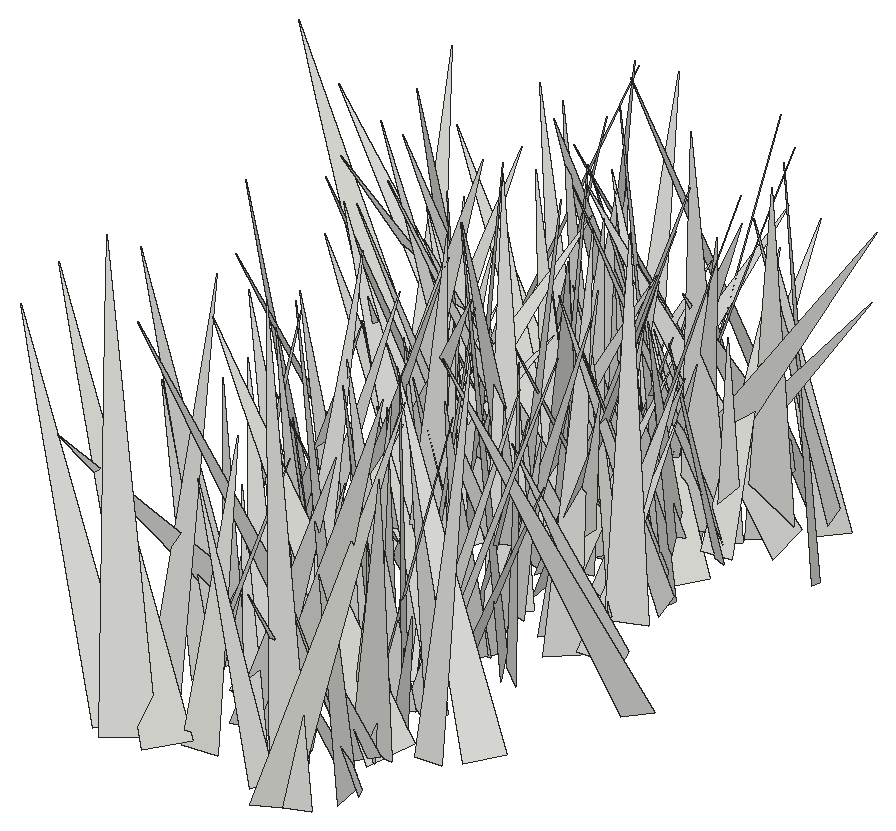
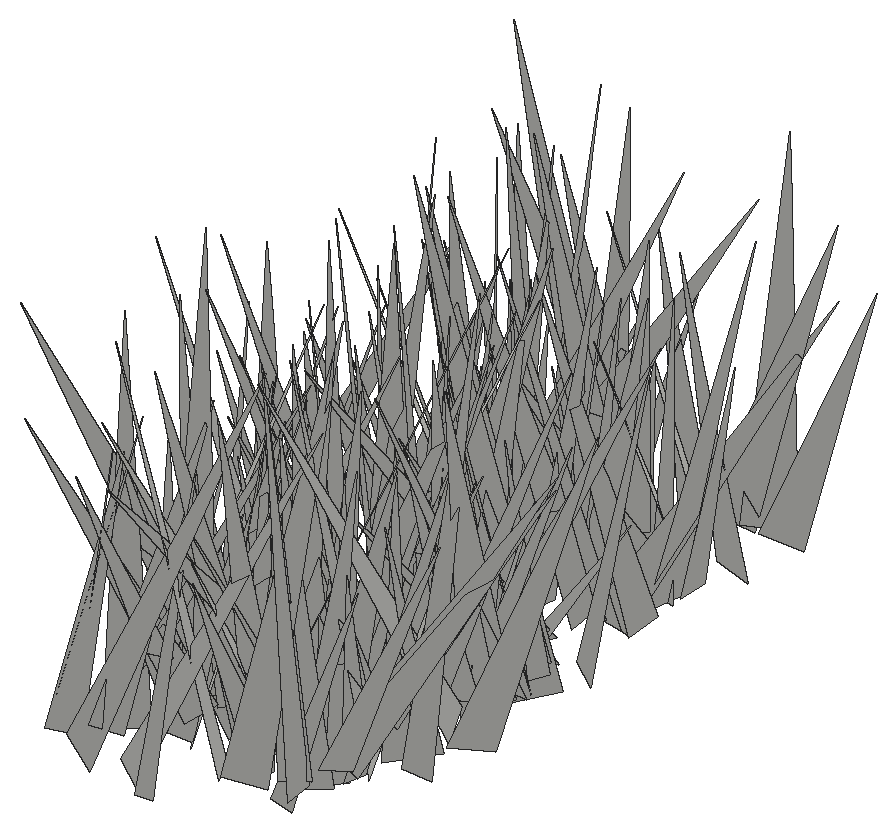
# SketchUp Ruby script. Lengths in inches.
U = 1.inch
M = Sketchup.active_model
def pt(a) = Geom::Point3d.new(a.map { |v| v * U })
def face(e, loops, mat)
  f = e.add_face(loops[0].map { |a| pt(a) })
  loops[1..].each { |l| e.add_face(l.map { |a| pt(a) }).erase! }
  f.material = f.back_material = mat if mat
  f
end
# faces: each face lists its corners as indices into pts; further lists are holes
def faces(e, pts, list, mat = nil) = list.each { |f| face(e, (f[0].is_a?(Array) ? f : [f]).map { |l| l.map { |i| pts[i] } }, mat) }
# xy, xz, yz: faces in a plane at the given z, y or x. An outline is a flat list of corners, or four numbers for a rectangle; further outlines are holes
def ring(l) = l.size == 4 ? [[l[0], l[1]], [l[2], l[1]], [l[2], l[3]], [l[0], l[3]]] : l.each_slice(2).to_a
def flat(e, list, mat, &to3) = list.each { |f| face(e, (f[0].is_a?(Array) ? f : [f]).map { |l| ring(l).map { |u, v| to3.(u, v) } }, mat) }
def xy(e, z, list, mat = nil) = flat(e, list, mat) { |x, y| [x, y, z] }
def xz(e, y, list, mat = nil) = flat(e, list, mat) { |x, z| [x, y, z] }
def yz(e, x, list, mat = nil) = flat(e, list, mat) { |y, z| [x, y, z] }
def lines(e, pts, list) = list.each { |a, b| e.add_line(pt(pts[a]), pt(pts[b])) }
# prism: a flat outline (further loops are holes) pulled along v
def prism(e, loops, v, mat = nil)
  f = face(e, loops, mat); d = Geom::Vector3d.new(v.map { |x| x * U })
  f.pushpull(f.normal.samedirection?(d) ? d.length : -d.length)
end
def box(e, o, s, mat = nil) = prism(e, [[o, [o[0] + s[0], o[1], o[2]], [o[0] + s[0], o[1] + s[1], o[2]], [o[0], o[1] + s[1], o[2]]]], [0, 0, s[2]], mat)
def at(x, y, z, deg = 0) = Geom::Transformation.translation(pt([x, y, z])) * Geom::Transformation.rotation(ORIGIN, Z_AXIS, deg.degrees)
def axes(o, x, y, z) = Geom::Transformation.new([*x, 0, *y, 0, *z, 0, *pt(o).to_a, 1])
def part(name) = M.definitions.add(name)
# library, detail: a bought-in or finely detailed component or shape, given as its bounding box
def library(name, o, s) = part(name).tap { |d| box(d.entities, o, s) }
def detail(e, o, s) = box(e.add_group.entities, o, s)
def put(e, d, t, mat = nil) = e.add_instance(d, t).tap { |i| i.material = mat if mat }
def group(e, t, mat = nil) = e.add_group.tap { |g| g.transformation = t; g.material = mat if mat }.entities
root = M.entities
c1 = part("fur_instance\#9")
p = [[0.8125,0,1.79],[0.67,-0.02,1.48],[0,-0.11,0],[0,0.11,0]]
faces(c1.entities,p,[[0,1,2,3]])
put(root,c1,axes([64.62,188,-27.1],[-5.80896,4.38047,0.69826],[4.41604,5.60261,1.59041],[-0.41794,-1.68592,7.09952]))
put(root,c1,axes([64.88,182.09,-27.1],[-3.28868,-4.79968,1.75844],[-5.10998,3.14053,-0.98472],[0.13097,2.01112,5.73434]))
put(root,c1,axes([66.55,170.2,-28.22],[-3.24359,5.98487,0.42852],[5.75195,2.96279,2.1587],[-1.708,-1.38792,6.45597]))
put(root,c1,axes([67.98,188.64,-27.1],[-5.05806,4.73106,0.08976],[4.36112,4.60989,2.7757],[-1.83619,-2.08349,6.34527]))
put(root,c1,axes([67.13,191.16,-27.1],[-0.73144,-5.99959,0.26703],[-5.39662,0.53861,-2.681],[-2.63493,0.56233,5.41685]))
put(root,c1,axes([67.08,191.65,-27.1],[-4.48303,2.72425,0.35571],[2.72908,4.33728,1.17718],[-0.3165,-1.18832,5.11208]))
put(root,c1,axes([66.97,175.47,-28.22],[-7.08698,0.49693,1.41438],[0.58095,7.2106,0.37757],[1.38199,-0.48283,7.09434]))
put(root,c1,axes([67.08,184.73,-27.1],[-4.89818,0.93846,0.55806],[1.01529,4.8584,0.74127],[0.40164,-0.83642,4.93188]))
put(root,c1,axes([68.67,170.12,-28.22],[-3.17251,7.14398,0.8627],[6.87917,2.73438,2.65436],[-2.11131,-1.82544,7.35225]))
put(root,c1,axes([66.78,174.3,-28.22],[-4.79431,0.50788,0.77321],[0.45097,4.84644,-0.38709],[0.80772,0.30866,4.80557]))
put(root,c1,axes([64.93,190.31,-27.1],[-2.27672,-7.40144,1.23154],[-7.29478,2.48469,1.44709],[1.75622,0.72557,7.60728]))
put(root,c1,axes([67.08,184.07,-28.22],[-6.50457,4.89284,0.5628],[4.72218,6.46057,-1.59001],[1.39918,0.94188,7.98255]))
put(root,c1,axes([67.36,186.7,-27.1],[-2.8111,-5.64649,0.53318],[-5.64839,2.7334,-0.83291],[-0.51273,0.84565,6.25232]))
put(root,c1,axes([68.09,181.38,-28.22],[-2.80536,-2.90649,0.0794],[-2.63209,2.49174,-1.78533],[-1.23535,1.29136,3.62358]))
put(root,c1,axes([67.5625,177.47,-28.22],[3.04305,-5.48081,0.27728],[-4.42438,-2.6378,-3.58374],[-3.24669,-1.54241,5.14356]))
put(root,c1,axes([67.4,169.73,-28.22],[-4.19179,6.94453,1.88873],[7.18228,4.17546,0.58769],[0.45687,-1.92457,8.09026]))
put(root,c1,axes([66.57,172.59,-28.22],[1.29784,6.7007,1.25957],[6.74597,-1.44798,0.75208],[-0.98888,-1.08363,6.78367]))
put(root,c1,axes([68.74,182.58,-28.22],[-2.83632,-6.0499,0.28173],[-5.90232,2.69141,-1.62612],[-1.35766,0.93829,6.48088]))
put(root,c1,axes([65.36,189.05,-27.1],[1.8239,-3.22944,0.77362],[-3.28665,-1.6292,0.94764],[0.47508,1.1273,3.58579]))
put(root,c1,axes([67.39,189.66,-28.22],[-3.97352,-3.33663,0.47318],[-3.25036,3.98768,0.8243],[0.89005,-0.33346,5.12275]))
put(root,c1,axes([67.52,190.17,-28.22],[-7.05336,-2.15617,1.71578],[-1.62887,7.06566,2.18314],[2.22256,-1.66441,7.04506]))
put(root,c1,axes([68.26,182.66,-27.1],[-3.16034,-1.96863,0.75138],[-2.10046,2.8354,-1.40585],[-0.16774,1.5852,3.44773]))
put(root,c1,axes([65.91,184.37,-27.1],[1.29367,6.30142,0.29631],[6.29029,-1.26564,-0.54746],[0.47747,-0.39942,6.4095]))
put(root,c1,axes([65.85,183.12,-27.1],[3.70802,-0.97097,0.29213],[-0.94384,-3.70994,-0.3508],[-0.37053,-0.26665,3.81695]))
put(root,c1,axes([67.24,175.28,-28.22],[1.09401,4.63876,2.44173],[5.21296,-1.22556,-0.00737],[-0.55243,-2.37843,4.76601]))
put(root,c1,axes([67.91,173.31,-28.22],[3.80784,5.11048,0.67094],[4.57882,-3.73693,2.47721],[-2.36675,0.99257,5.87197]))
put(root,c1,axes([68.39,189.01,-28.22],[-4.24883,1.88722,0.42776],[1.75815,4.19597,-1.04876],[0.80838,0.79335,4.52927]))
put(root,c1,axes([66.7,185.7,-27.1],[1.07751,-3.9043,2.33703],[-4.53898,-0.75293,0.83488],[0.32078,2.46086,3.96327]))
put(root,c1,axes([68.27,192.88,-28.22],[-0.08918,-3.86635,0.81214],[-3.84672,-0.10019,-0.89937],[-0.90053,0.81086,3.76135]))
put(root,c1,axes([68.89,176.65,-28.22],[-2.59565,5.50063,1.7013],[5.74289,2.3395,1.19781],[-0.41302,-2.03926,5.96319]))
put(root,c1,axes([65.99,187.07,-27.1],[6.85876,3.23862,0.41321],[3.02392,-6.66397,2.03701],[-1.23097,1.67477,7.30628]))
put(root,c1,axes([69.88,189.02,-28.22],[-6.64184,2.29308,0.28161],[2.23011,6.58737,-1.04152],[0.60342,0.8944,6.94892]))
put(root,c1,axes([67.77,188.22,-28.22],[1.11267,-4.69864,0.20362],[-4.67497,-1.12782,-0.47895],[-0.51316,0.0867,4.80478]))
put(root,c1,axes([69.62,184.96,-27.1],[-4.99004,2.24313,0.58277],[2.2784,5.00139,0.2583],[0.42444,-0.4756,5.46492]))
put(root,c1,axes([68.89,185,-27.1],[-3.32365,-1.7064,1.24939],[-2.04417,3.18881,-1.08271],[0.54234,1.56176,3.57578]))
put(root,c1,axes([67.33,184.88,-27.1],[4.65411,-4.15615,0.09318],[-4.0063,-4.52139,-1.56511],[-1.10988,-1.10744,6.04026]))
put(root,c1,axes([67.25,188.45,-28.22],[4.72712,-1.54603,0.79765],[-1.39638,-4.74943,-0.93014],[-1.03759,-0.65178,4.88576]))
put(root,c1,axes([66.54,177.04,-28.22],[6.22243,-0.20354,0.93497],[-0.30289,-6.25415,0.65425],[-0.90767,0.69164,6.19128]))
put(root,c1,axes([69.18,176.63,-28.22],[4.90342,0.51596,3.18153],[0.4361,-5.84514,0.27581],[-3.19346,-0.00597,4.92277]))
put(root,c1,axes([67.07,193.55,-27.1],[6.76883,1.43904,1.95286],[1.74836,-6.90673,-0.9705],[-1.68159,-1.38844,6.85171]))
put(root,c1,axes([66.41,183.87,-27.1],[-0.23722,4.19444,0.05409],[3.55446,0.22976,-2.22834],[2.22756,0.08005,3.56147]))
put(root,c1,axes([67.0625,182.21,-28.22],[3.97347,4.57155,1.31094],[4.73936,-3.94824,-0.59665],[-0.39506,-1.38509,6.02757]))
put(root,c1,axes([71.19,183.9,-27.1],[-7.48937,-0.81173,0.36322],[-0.84224,7.4632,-0.68756],[0.28542,0.72333,7.50179]))
put(root,c1,axes([67.51,180.82,-28.22],[-0.63862,5.35473,0.03552],[5.1577,0.62471,-1.44573],[1.43964,0.13724,5.19527]))
put(root,c1,axes([67.02,189.9375,-27.1],[6.14666,2.4589,1.36982],[2.59506,-6.2248,-0.47069],[-1.09008,-0.95377,6.60349]))
put(root,c1,axes([69.4,183.05,-27.1],[-4.06626,4.25963,1.22614],[4.27905,4.20638,-0.4224],[1.15655,-0.5867,5.87371]))
put(root,c1,axes([69.06,184.62,-28.22],[-4.34525,-4.69158,2.51984],[-5.05188,4.66036,-0.03462],[1.68493,1.87398,6.3946]))
put(root,c1,axes([67.78,190.75,-28.22],[4.73789,-1.18845,0.72275],[-0.9672,-4.65874,-1.32025],[-0.99966,-1.12521,4.70287]))
put(root,c1,axes([70.86,186.67,-28.22],[-3.00084,5.06154,0.45444],[5.0055,2.85272,1.2797],[-0.87785,-1.03611,5.74339]))
put(root,c1,axes([69.875,178.06,-28.22],[-6.22894,0.57755,1.75246],[0.68588,6.45268,0.31131],[1.71297,-0.48351,6.24791]))
put(root,c1,axes([67.48,177.55,-28.22],[2.77668,6.00015,1.42785],[6.14966,-2.57364,-1.14395],[0.47149,-1.76779,6.51177]))
put(root,c1,axes([66.7,182.66,-27.1],[0.11593,7.32982,3.76994],[7.80213,1.11829,-2.4142],[2.6581,-3.60212,6.9218]))
put(root,c1,axes([70.47,187.62,-27.1],[2.04194,-5.37013,1.21962],[-4.97283,-2.35693,-2.05211],[-2.36574,0.31918,5.36625]))
put(root,c1,axes([67.66,192.96,-27.1],[0.9975,-5.62203,0.93729],[-5.55991,-0.75041,1.41599],[1.25425,1.14473,5.53148]))
put(root,c1,axes([68.82,194.03,-27.1],[1.6119,-7.35068,0.1441],[-7.34568,-1.61634,-0.28263],[-0.30696,0.08011,7.52003]))
put(root,c1,axes([68.14,191.46,-28.22],[2.75053,-5.09352,1.52718],[-5.31748,-2.64324,0.76119],[-0.02665,1.70616,5.73847]))
put(root,c1,axes([70.69,185.05,-28.22],[-0.44719,-4.16584,0.88919],[-4.01944,0.11666,-1.47491],[-1.41032,0.98845,3.92158]))
put(root,c1,axes([69.04,176.18,-28.22],[-1.25475,3.57203,1.31412],[3.70812,1.4592,-0.42579],[0.858,-1.08261,3.76198]))
put(root,c1,axes([67.28,181.39,-27.1],[-1.44675,6.62808,0.1342],[5.91861,1.35324,-3.03008],[2.98656,0.529,6.06986]))
put(root,c1,axes([68.09,185.27,-28.22],[3.1539,-2.32332,0.00557],[-2.32207,-3.15188,0.13648],[0.07647,0.11319,3.91488]))
put(root,c1,axes([70.49,172.875,-28.22],[3.00603,-4.02582,3.59921],[-4.80148,-3.87769,-0.32715],[-2.47129,2.63706,5.01362]))
put(root,c1,axes([70.3125,186.72,-28.22],[-1.93771,-4.14246,0.35212],[-4.15628,1.93921,-0.05843],[0.0961,0.34375,4.57288]))
put(root,c1,axes([72.51,182.65,-27.1],[-6.31151,-2.93767,0.11387],[-2.9284,6.25835,-0.85765],[-0.25951,0.82534,6.90866]))
put(root,c1,axes([69.65,170.5,-28.22],[-1.16882,5.10436,1.64073],[5.31118,1.33199,-0.3603],[0.7334,-1.51127,5.22406]))
put(root,c1,axes([71.24,171.35,-28.22],[-0.27528,4.26527,0.41219],[4.05575,0.12601,1.40472],[-1.38323,-0.47937,4.03672]))
put(root,c1,axes([71.03,186.8125,-27.1],[-1.86081,5.49202,1.44787],[5.66351,1.67938,0.90859],[-0.42807,-1.65488,5.72707]))
put(root,c1,axes([68.9375,176.53,-28.22],[1.7878,3.1828,1.34143],[3.44443,-1.53093,-0.95817],[0.2561,-1.62848,3.52255]))
put(root,c1,axes([74.05,173.3125,-28.22],[-3.051,-7.21191,1.32168],[-6.61753,2.09219,-3.8598],[-3.15701,2.58422,6.81338]))
put(root,c1,axes([72.47,179.52,-28.22],[-6.11884,4.72961,1.11538],[4.85918,5.97068,1.339],[0.0418,-1.7422,7.61686]))
put(root,c1,axes([68.74,173.93,-28.22],[-1.28039,5.01222,0.36244],[4.5705,1.31696,-2.06622],[2.08908,0.19072,4.74262]))
put(root,c1,axes([70.63,180.96,-28.22],[-4.7564,-0.43454,1.78324],[-0.95829,4.81251,-1.3833],[1.56539,1.62573,4.5715]))
put(root,c1,axes([66.38,182.54,-28.22],[3.10816,-7.62871,0.22312],[-7.12075,-2.81203,3.04879],[2.74626,1.34273,7.65263]))
put(root,c1,axes([70.68,175.83,-28.22],[3.31439,2.62679,2.62231],[3.03004,-3.94532,0.12232],[-2.14367,-1.5153,4.22732]))
put(root,c1,axes([69.23,184.2,-28.22],[6.90611,3.10223,2.59996],[3.46907,-7.18559,-0.64093],[-2.08547,-1.6797,7.5437]))
put(root,c1,axes([68.28,171.6,-28.22],[4.70564,3.18962,0.73071],[3.27223,-4.59158,-1.02983],[-0.01227,-1.26267,5.59072]))
put(root,c1,axes([68.32,177.56,-28.22],[7.58645,0.4489,1.20084],[0.2907,-7.62155,1.01257],[-1.24861,0.95304,7.53196]))
put(root,c1,axes([70.88,190.52,-27.1],[-0.70792,6.63222,0.94241],[6.69223,0.65809,0.39581],[-0.29764,-0.97786,6.65814]))
put(root,c1,axes([72.08,187.16,-27.1],[-6.95078,-0.2098,1.40903],[-0.48679,6.94525,-1.36721],[1.33881,1.43604,6.81821]))
put(root,c1,axes([70.14,191.64,-28.22],[3.6116,-2.54944,1.03868],[-2.46348,-3.75778,-0.65768],[-1.22872,0.0404,4.37159]))
put(root,c1,axes([70.62,190.91,-28.22],[-2.94733,3.27814,0.42411],[3.06608,2.92358,-1.29021],[1.23501,0.56503,4.21525]))
put(root,c1,axes([68.83,190.6,-27.1],[1.67584,3.97009,0.12724],[3.80521,-1.56498,-1.28741],[1.13936,-0.61275,4.1125]))
put(root,c1,axes([72.51,170.03,-28.22],[-4.9286,0.63717,0.02707],[0.62924,4.89286,-0.60144],[0.10377,0.59304,4.93308]))
put(root,c1,axes([71.65,180.29,-28.22],[0.78619,5.10987,0.99795],[4.99569,-1.02461,1.31074],[-1.46621,-0.75112,5.00108]))
put(root,c1,axes([73.25,185.13,-27.1],[-6.90561,-3.33755,0.10935],[-3.32242,6.89219,0.54573],[0.33571,-0.44394,7.65042]))
put(root,c1,axes([73.2,194.27,-28.22],[-3.69679,-5.87263,0.02895],[-5.78236,3.6339,-1.23044],[-1.02613,0.67962,6.82936]))
put(root,c1,axes([71.11,177.5625,-28.22],[-3.39336,2.50243,2.08506],[2.97495,3.60715,0.51243],[1.32637,-1.68843,4.18502]))
put(root,c1,axes([71.59,190.17,-28.22],[-4.44345,-1.97155,1.25823],[-1.71315,4.58269,1.13072],[1.59225,-0.57131,4.72787]))
put(root,c1,axes([71.38,189.24,-28.22],[3.36886,3.17868,0.5186],[2.75759,-3.23451,1.91201],[-1.66392,1.0752,4.2187]))
put(root,c1,axes([74.49,173.95,-28.22],[-6.95314,3.37085,0.59923],[3.40426,6.66259,2.02209],[-0.36434,-2.07731,7.45788]))
put(root,c1,axes([68.25,187.45,-28.22],[3.98085,5.13777,1.04709],[4.9615,-3.26572,-2.83883],[1.69606,-2.50573,5.84679]))
put(root,c1,axes([70.56,186.32,-28.22],[-0.53064,3.51066,0.60828],[3.36851,0.69471,-1.0709],[1.16098,-0.41106,3.38519]))
put(root,c1,axes([73.09,178.31,-28.22],[-4.19942,1.95994,0.17006],[1.96728,4.18576,0.33862],[0.01038,-0.37878,4.62189]))
put(root,c1,axes([70.54,188.29,-28.22],[3.92094,-4.8226,1.73149],[-5.06492,-3.97791,0.39007],[-0.77596,1.59628,6.20315]))
put(root,c1,axes([71.25,186.01,-28.22],[4.78863,4.89843,2.46119],[5.13986,-5.14824,0.24599],[-1.90629,-1.57608,6.84581]))
put(root,c1,axes([72.375,178.27,-28.22],[-2.92778,3.00983,0.00711],[2.98882,2.90849,-0.48849],[0.35507,0.33555,4.17041]))
put(root,c1,axes([73.11,191.22,-28.22],[-5.49942,-3.45806,0.94275],[-3.51329,5.5426,-0.16378],[0.70973,0.64178,6.49422]))
put(root,c1,axes([71.97,189.28,-27.1],[2.76185,-3.07557,2.49035],[-3.57907,-3.23702,-0.02845],[-1.68858,1.83068,4.13354]))
put(root,c1,axes([70.5,189.77,-27.1],[2.46707,-3.42013,1.11602],[-3.59628,-2.30764,0.87798],[0.09798,1.4166,4.12467]))
put(root,c1,axes([71.31,184.68,-27.1],[-1.28259,-7.19659,1.19017],[-7.23451,1.40948,0.72639],[0.93233,1.03678,7.27381]))
put(root,c1,axes([71.2,179.47,-28.22],[6.01123,-4.10409,2.83515],[-4.50522,-6.3728,0.32708],[-2.14119,1.8869,7.27128]))
put(root,c1,axes([72.04,181.125,-28.22],[-1.26664,-5.03308,1.07763],[-5.14261,1.28411,-0.04714],[0.2163,1.05675,5.1898]))
put(root,c1,axes([72.18,171.66,-28.22],[0.64716,8.27924,1.09317],[8.31403,-0.74193,0.69715],[-0.78591,-1.0312,8.27518]))
put(root,c1,axes([71.83,186.15,-27.1],[1.95949,2.80373,1.45551],[3.04239,-2.136,0.01872],[-0.85045,-1.18135,3.42055]))
put(root,c1,axes([71.94,179.45,-28.22],[-1.89592,-3.45095,1.30694],[-3.60556,2.04518,0.16982],[0.78554,1.05823,3.9338]))
put(root,c1,axes([69.42,188.66,-28.22],[7.63705,-2.12328,0.08153],[-2.0044,-7.29978,-2.35267],[-0.70524,-2.24596,7.56953]))
put(root,c1,axes([71.75,177.41,-28.22],[-2.18081,-4.36379,1.96245],[-4.63729,2.45895,0.31456],[1.17875,1.60022,4.86823]))
put(root,c1,axes([72.92,181.76,-27.1],[-5.4488,4.52209,1.619],[4.59694,5.6194,-0.22458],[1.39234,-0.85616,7.07731]))
put(root,c1,axes([70.47,187.34,-28.22],[-3.50989,5.55769,0.51718],[4.45011,3.15505,-3.70364],[3.36927,1.62248,5.4305]))
put(root,c1,axes([70.01,172.62,-28.22],[3.9818,-4.86666,0.84742],[-4.90357,-3.76221,1.43455],[0.59785,1.55519,6.12218]))
put(root,c1,axes([70.375,189.55,-28.22],[4.5818,0.64032,0.1617],[0.65902,-4.5067,-0.82732],[-0.04299,-0.84188,4.55176]))
put(root,c1,axes([71.02,184.37,-28.22],[-4.14785,-5.45032,3.6874],[-5.74845,5.12259,1.10541],[3.20285,2.13555,6.75935]))
put(root,c1,axes([72.76,176.3125,-28.22],[1.22573,-5.85041,2.29876],[-6.17569,-1.55733,-0.67049],[-1.1715,2.08841,5.93971]))
put(root,c1,axes([72.17,189.46,-28.22],[2.53184,-2.74895,1.13947],[-2.76231,-2.72751,-0.44237],[-1.1067,0.51894,3.71097]))
put(root,c1,axes([74.16,169.38,-28.22],[0.0482,8.00911,1.76337],[7.92916,-0.49572,2.03478],[-2.09374,-1.69294,7.74648]))
put(root,c1,axes([74.1,176.71,-28.22],[-5.98582,-0.44068,0.88109],[-0.67667,5.78235,-1.70504],[0.71598,1.78068,5.75475]))
put(root,c1,axes([71.77,178.54,-28.22],[-4.21577,-3.58718,3.5566],[-4.31781,4.96325,-0.11214],[2.62178,2.40587,5.53425]))
put(root,c1,axes([75.28,194.2,-28.22],[-3.74944,-6.99723,1.04952],[-6.92154,3.38084,-2.18706],[-1.468,1.93125,7.63127]))
put(root,c1,axes([74.86,188.21,-28.22],[-5.62336,3.63446,0.06059],[3.63174,5.6129,0.37548],[-0.15301,-0.3482,6.6851]))
put(root,c1,axes([71.91,195.17,-28.22],[-1.799,-4.93024,0.4482],[-4.7112,1.85147,1.45641],[1.52075,-0.09654,5.04207]))
put(root,c1,axes([75.29,186.84,-28.22],[-7.24108,-2.76695,1.69952],[-3.23599,6.49389,-3.21487],[0.2698,3.62643,7.05364]))
put(root,c1,axes([72.39,176.3,-28.22],[-2.8459,-6.01928,1.64103],[-5.98512,3.14324,1.14988],[1.76154,0.95508,6.5581]))
put(root,c1,axes([71.13,192.23,-28.22],[6.44327,3.68852,1.42181],[3.82977,-6.4983,-0.49739],[-0.97955,-1.14429,7.40767]))
put(root,c1,axes([70.53,191.41,-27.1],[4.49175,-3.99144,0.42922],[-3.97143,-4.32409,1.3497],[0.58618,1.28931,5.8554]))
put(root,c1,axes([73.4,191.49,-28.22],[0.72019,-3.80208,0.86926],[-3.795,-0.88705,-0.73566],[-0.89965,0.69817,3.79912]))
put(root,c1,axes([74.04,187.76,-28.22],[-0.0394,4.36961,1.02441],[4.32756,-0.23455,1.1669],[-1.18959,-0.99797,4.2111]))
put(root,c1,axes([72.4,180.65,-28.22],[1.15457,-5.41906,0.82486],[-5.48032,-1.12384,0.28761],[0.11275,0.86626,5.53322]))
put(root,c1,axes([74.7,185.91,-27.1],[-2.68226,-4.58353,0.12394],[-4.53778,2.63294,-0.83358],[-0.65781,0.52677,5.24485]))
put(root,c1,axes([75.77,192.05,-28.22],[-7.08449,-0.21202,0.14595],[-0.16992,6.87165,1.73429],[0.19334,-1.72965,6.8722]))
put(root,c1,axes([74.17,172.25,-28.22],[-0.70477,-3.63934,0.22038],[-3.52996,0.62491,-0.96896],[-0.91253,0.39339,3.57807]))
put(root,c1,axes([72.28,182.85,-27.1],[3.06057,-3.28635,0.3748],[-3.27189,-3.08287,-0.31361],[-0.4851,0.05914,4.47983]))
put(root,c1,axes([73.59,183.02,-28.22],[4.93577,0.48548,2.66433],[-0.37318,-5.36398,1.66873],[-2.68236,1.63958,4.67042]))
put(root,c1,axes([71.99,176.32,-28.22],[5.04239,2.3615,1.06864],[2.46365,-5.09289,-0.37039],[-0.80566,-0.79378,5.55564]))
put(root,c1,axes([75.08,171.04,-28.22],[-7.60319,-2.30719,2.08818],[-2.71089,7.61771,-1.45385],[1.52798,2.03457,7.8114]))
put(root,c1,axes([73.71,180.53,-28.22],[-6.4664,-4.252,2.80304],[-4.40658,6.94256,0.3657],[2.55316,1.21333,7.73047]))
put(root,c1,axes([71.67,181.52,-28.22],[5.00049,1.26706,0.71261],[1.41038,-4.84715,-1.27832],[-0.35226,-1.4205,4.99762]))
put(root,c1,axes([72.71,176.88,-28.22],[5.57047,2.74276,2.66238],[3.42235,-5.67452,-1.31471],[-1.7025,-2.43273,6.06831]))
put(root,c1,axes([72.92,188.58,-27.1],[5.4592,3.52611,0.65952],[3.05756,-5.20187,2.50265],[-1.87611,1.78282,5.99776]))
put(root,c1,axes([73.09,174.9,-28.22],[2.3019,2.88607,2.09295],[3.52279,-2.224,-0.8077],[-0.54756,-2.17555,3.60219]))
put(root,c1,axes([72.22,184.58,-27.1],[6.79493,0.95964,1.40947],[0.56386,-6.72962,1.86359],[-1.60922,1.6941,6.60447]))
put(root,c1,axes([73.84,187.9,-28.22],[-0.71572,-3.67555,0.46048],[-3.70429,0.70984,-0.09154],[-0.00255,0.46948,3.74347]))
put(root,c1,axes([75.4375,189.53,-27.1],[-5.5722,-4.07145,0.43281],[-4.071,5.58734,0.1482],[0.43699,0.13539,6.89957]))
put(root,c1,axes([72.9,186.29,-27.1],[4.01633,-1.15722,1.23996],[-1.33038,-4.12648,0.45808],[-1.05202,0.80037,4.15454]))
put(root,c1,axes([74.7,182.19,-28.22],[-6.34351,2.24327,1.15963],[1.89857,6.30395,-1.80908],[1.66506,1.35834,6.48071]))
put(root,c1,axes([72.1875,190.47,-27.1],[2.06201,-3.51619,0.27094],[-3.44771,-1.94389,1.0117],[0.74186,0.73932,3.94867]))
put(root,c1,axes([72.89,180.71,-28.22],[5.70541,0.17051,1.69377],[-0.31532,-5.71566,1.63753],[-1.67287,1.65887,5.46803]))
put(root,c1,axes([75.24,171.5,-28.22],[-3.08913,-1.9262,0.20442],[-1.91689,2.98464,-0.84391],[-0.27849,0.82245,3.5413]))
put(root,c1,axes([72.55,189.52,-27.1],[3.14021,-1.95272,0.11029],[-1.95573,-3.13292,0.21476],[0.01996,0.24059,3.6916]))
put(root,c1,axes([72.22,187.86,-28.22],[2.89103,-3.61881,0.35286],[-3.55779,-2.72252,1.22815],[0.74997,1.03461,4.46604]))
put(root,c1,axes([73.18,176.8,-28.22],[3.13584,4.70476,0.63652],[4.72939,-3.16238,0.0748],[-0.41563,-0.48786,5.65355]))
put(root,c1,axes([73.07,181.78,-27.1],[0.44262,-3.83329,1.02735],[-3.85493,-0.16968,1.02773],[0.94293,1.1057,3.71938]))
put(root,c1,axes([71.35,172.6,-28.22],[3.88235,-7.18309,1.19208],[-7.15051,-3.50623,2.16032],[1.37403,2.04942,7.87416]))
put(root,c1,axes([73.09,185.1,-27.1],[1.90373,-3.64825,0.45227],[-3.65968,-1.83258,0.622],[0.34793,0.68584,4.0678]))
put(root,c1,axes([75.74,183.69,-27.1],[-4.50739,-0.00087,0.31518],[-0.09503,4.31184,-1.34718],[0.30051,1.35052,4.30136]))
put(root,c1,axes([72.86,179.42,-28.22],[4.07736,0.20577,0.16386],[0.20057,-4.0788,0.13116],[-0.17019,0.12285,4.08044]))
put(root,c1,axes([73.63,173.57,-28.22],[2.13967,5.72529,2.72362],[6.33838,-1.99885,-0.77766],[-0.14822,-2.82858,6.06237]))
put(root,c1,axes([76.92,175.6,-28.22],[-4.13597,4.87198,0.25098],[4.78591,3.98836,1.44689],[-0.94567,-1.12348,6.22487]))
put(root,c1,axes([73.26,184.18,-27.1],[1.23248,3.89294,0.26564],[3.83774,-1.15903,-0.82034],[0.70519,-0.49622,4.00013]))
put(root,c1,axes([74.26,194.09,-27.1],[4.06405,-3.6671,0.18626],[-3.28339,-3.75381,-2.26428],[-1.64366,-1.56845,4.98369]))
put(root,c1,axes([73.89,191.07,-27.1],[-1.59492,4.69203,0.53683],[4.53057,1.68008,-1.22409],[1.33316,-0.09626,4.80214]))
put(root,c1,axes([73.97,188.83,-28.22],[3.35364,-3.87615,0.32814],[-3.76663,-3.34394,-1.00479],[-0.97195,-0.41544,5.02611]))
put(root,c1,axes([74.29,180.17,-28.22],[-3.23296,-4.09809,2.47034],[-4.47809,3.64184,0.18098],[1.68632,1.81429,5.21667]))
put(root,c1,axes([75.4375,186.47,-27.1],[-3.54687,-2.63553,0.56126],[-2.61948,3.58991,0.30355],[0.63194,0.08835,4.40842]))
put(root,c1,axes([72.86,183.51,-27.1],[6.72772,1.76518,0.89994],[1.69777,-6.77807,0.60273],[-1.02144,0.36032,6.92927]))
put(root,c1,axes([73.64,169.1,-28.22],[6.32729,-2.1008,2.73388],[-3.01636,-6.1404,2.26257],[-1.67006,3.13117,6.27127]))
put(root,c1,axes([74.49,189.54,-27.1],[2.05152,-6.96349,2.48946],[-7.36809,-2.14532,0.07104],[-0.63146,2.40909,7.25905]))
put(root,c1,axes([75.61,174.39,-28.22],[1.51119,6.34193,0.92742],[6.21067,-1.68435,1.39797],[-1.58356,-0.55387,6.36784]))
put(root,c1,axes([73.45,190.47,-27.1],[0.26156,-6.27199,1.2943],[-6.21893,0.06053,1.55008],[1.52905,1.31908,6.08306]))
put(root,c1,axes([76.52,185.09,-27.1],[-5.39834,-1.72938,0.70035],[-1.70183,5.44274,0.32197],[0.76486,-0.09564,5.65943]))
put(root,c1,axes([76.01,188.375,-27.1],[-2.1087,-2.96786,0.97974],[-3.12443,1.97245,-0.74971],[-0.07759,1.23123,3.56269]))
put(root,c1,axes([73.56,176.65,-28.22],[4.96936,4.425,0.65774],[4.44372,-4.99597,0.03757],[-0.51632,-0.4092,6.65385]))
put(root,c1,axes([73.96,188.97,-28.22],[5.97611,0.87511,2.00016],[1.66713,-5.59279,-2.53411],[-1.40966,-2.90435,5.48252]))
put(root,c1,axes([73.98,173.64,-28.22],[1.6892,-5.96403,1.00433],[-6.01842,-1.55459,0.89085],[0.59746,1.20222,6.13428]))
put(root,c1,axes([73.14,186.63,-27.1],[6.72571,2.73267,0.89443],[2.78268,-6.75899,-0.27437],[-0.72399,-0.59256,7.25447]))
put(root,c1,axes([73.93,175.08,-28.22],[-0.71595,-3.844,0.50308],[-3.36107,0.87042,1.86752],[1.93201,0.08975,3.4353]))
put(root,c1,axes([75.72,188.58,-27.1],[-0.62554,4.99616,0.12365],[4.99768,0.62512,0.02455],[-0.009,-0.12574,5.03511]))
put(root,c1,axes([75.35,182.7,-28.22],[-2.96386,2.60362,0.59977],[2.15648,2.85999,-1.75873],[1.5774,0.98217,3.53132]))
put(root,c1,axes([76.49,193.4375,-28.22],[2.18952,-4.24382,2.13551],[-4.35668,-2.73133,-0.96101],[-1.89466,1.3763,4.67766]))
put(root,c1,axes([75.52,189.48,-27.1],[2.21811,-2.97156,1.30139],[-3.14682,-2.35396,-0.01147],[-0.78819,1.03561,3.7081]))
put(root,c1,axes([76.21,183.51,-27.1],[-2.20554,5.93145,2.00046],[6.2413,2.24627,0.22087],[0.47966,-1.95462,6.32437]))
put(root,c1,axes([75.07,192.0625,-28.22],[4.72126,-4.87179,1.88096],[-5.03873,-4.91595,-0.08523],[-1.37242,1.28908,6.78361]))
put(root,c1,axes([78.01,190.66,-28.22],[-6.09623,-2.24198,1.5344],[-2.70516,5.35755,-2.91953],[0.25098,3.28863,5.80232]))
put(root,c1,axes([77.05,192.76,-27.1],[-4.90354,-1.85753,0.89414],[-1.8937,4.97041,-0.05944],[0.81474,0.37312,5.24324]))
put(root,c1,axes([72.56,191.47,-27.1],[3.74419,-3.98525,0.35569],[-3.51637,-3.04515,2.89653],[1.90889,2.20738,4.63803]))
put(root,c1,axes([74.67,184.33,-27.1],[-0.11814,4.24138,1.60816],[4.31681,0.59918,-1.26317],[1.39308,-1.49704,4.05064]))
put(root,c1,axes([76.49,182.91,-28.22],[-4.80536,-1.45342,1.08645],[-0.98448,4.67157,1.89512],[1.52434,-1.5647,4.64891]))
put(root,c1,axes([72.05,189.53,-28.22],[5.69226,-5.26322,0.96159],[-5.00885,-4.7486,3.65927],[1.88086,3.28288,6.8347]))
put(root,c1,axes([78.88,180.75,-28.22],[-0.65869,-6.64833,1.3688],[-6.16249,0.00919,-2.92087],[-2.84565,1.51902,6.00855]))
